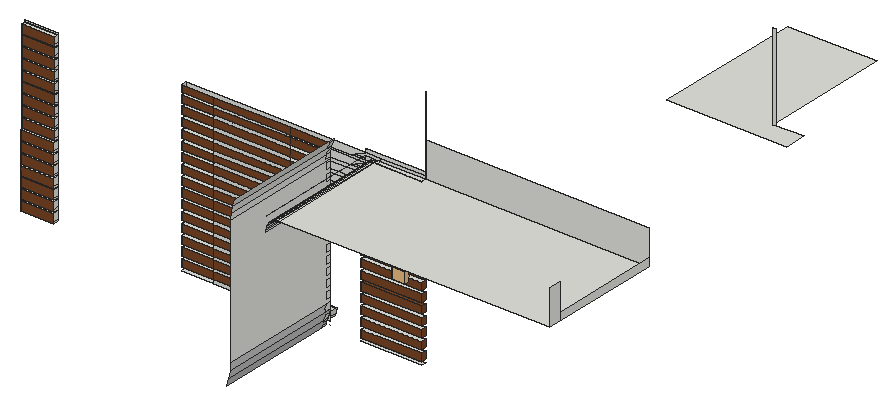
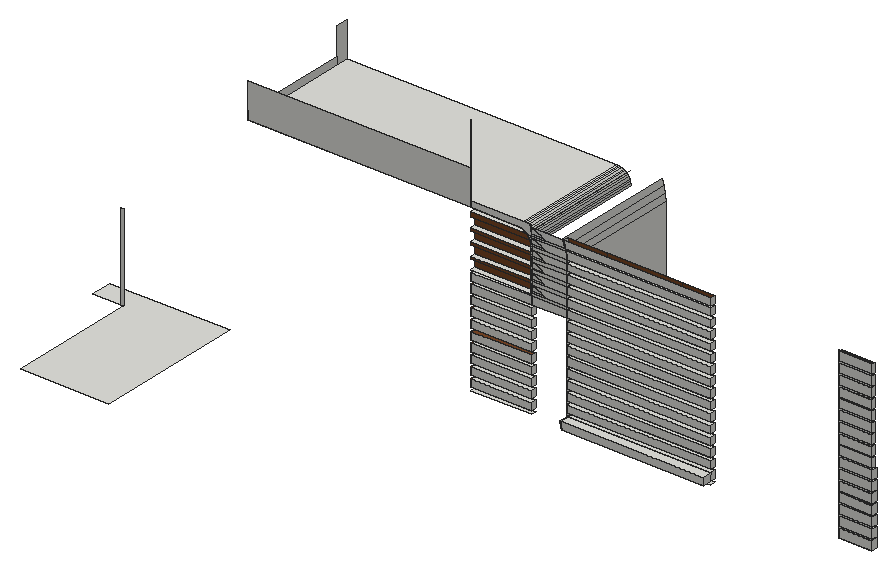
# SketchUp Ruby script. Lengths in inches.
U = 1.inch
M = Sketchup.active_model
def pt(a) = Geom::Point3d.new(a.map { |v| v * U })
def face(e, loops, mat)
  f = e.add_face(loops[0].map { |a| pt(a) })
  loops[1..].each { |l| e.add_face(l.map { |a| pt(a) }).erase! }
  f.material = f.back_material = mat if mat
  f
end
# faces: each face lists its corners as indices into pts; further lists are holes
def faces(e, pts, list, mat = nil) = list.each { |f| face(e, (f[0].is_a?(Array) ? f : [f]).map { |l| l.map { |i| pts[i] } }, mat) }
# xy, xz, yz: faces in a plane at the given z, y or x. An outline is a flat list of corners, or four numbers for a rectangle; further outlines are holes
def ring(l) = l.size == 4 ? [[l[0], l[1]], [l[2], l[1]], [l[2], l[3]], [l[0], l[3]]] : l.each_slice(2).to_a
def flat(e, list, mat, &to3) = list.each { |f| face(e, (f[0].is_a?(Array) ? f : [f]).map { |l| ring(l).map { |u, v| to3.(u, v) } }, mat) }
def xy(e, z, list, mat = nil) = flat(e, list, mat) { |x, y| [x, y, z] }
def xz(e, y, list, mat = nil) = flat(e, list, mat) { |x, z| [x, y, z] }
def yz(e, x, list, mat = nil) = flat(e, list, mat) { |y, z| [x, y, z] }
def lines(e, pts, list) = list.each { |a, b| e.add_line(pt(pts[a]), pt(pts[b])) }
# prism: a flat outline (further loops are holes) pulled along v
def prism(e, loops, v, mat = nil)
  f = face(e, loops, mat); d = Geom::Vector3d.new(v.map { |x| x * U })
  f.pushpull(f.normal.samedirection?(d) ? d.length : -d.length)
end
def box(e, o, s, mat = nil) = prism(e, [[o, [o[0] + s[0], o[1], o[2]], [o[0] + s[0], o[1] + s[1], o[2]], [o[0], o[1] + s[1], o[2]]]], [0, 0, s[2]], mat)
def at(x, y, z, deg = 0) = Geom::Transformation.translation(pt([x, y, z])) * Geom::Transformation.rotation(ORIGIN, Z_AXIS, deg.degrees)
def axes(o, x, y, z) = Geom::Transformation.new([*x, 0, *y, 0, *z, 0, *pt(o).to_a, 1])
def part(name) = M.definitions.add(name)
# library, detail: a bought-in or finely detailed component or shape, given as its bounding box
def library(name, o, s) = part(name).tap { |d| box(d.entities, o, s) }
def detail(e, o, s) = box(e.add_group.entities, o, s)
def put(e, d, t, mat = nil) = e.add_instance(d, t).tap { |i| i.material = mat if mat }
def group(e, t, mat = nil) = e.add_group.tap { |g| g.transformation = t; g.material = mat if mat }.entities
root = M.entities
M.materials.add("[Color M02]").color = [198, 198, 198]
M.materials.add("[Wood Veneer 01]").color = [120, 70, 37]
c1 = library("Spot+Bela",[0,3.21,0],[8.99,3.48,7.7])
xy(root,84.625,[[338.58,345.98,352.5,348.1]])
xy(root,85.73,[[405.46,345.98,463.86,348.1],[480.01,345.98,505.26,348.1]])
xy(root,87.0625,[[405.46,345.98,464.3125,348.1],[480.01,345.98,505.26,348.1],[405.46,348.1,464.3125,352.04]])
xy(root,88.34,[[338.58,345.98,352.5,348.1]])
xy(root,89,[[338.58,345.98,352.5,348.1]])
xy(root,90.11,[[405.46,345.98,465.05,348.1],[480.01,345.98,505.26,348.1],[405.46,348.1,465.05,352.04]])
xy(root,91.45,[[405.46,345.98,465.27,348.1],[480.01,345.98,505.26,348.1]])
xy(root,92.72,[[338.58,345.98,352.5,348.1]])
xy(root,93.375,[[338.58,345.98,352.5,348.1]])
xy(root,94.5,[[405.46,345.98,465.45,348.1],[480.01,345.98,505.26,348.1]])
xy(root,95.83,[[405.46,345.98,465.45,348.1],[480.01,345.98,505.26,348.1]])
xy(root,97.09,[[338.58,345.98,352.5,348.1]])
xy(root,97.75,[[338.58,345.98,352.5,348.1]])
xy(root,98.88,[[405.46,345.98,465.45,348.1],[480.01,345.98,505.26,348.1]])
xy(root,100.22,[[405.46,345.98,465.45,348.1],[480.01,345.98,505.26,348.1]])
xy(root,101.47,[[338.58,345.98,352.5,348.1]])
xy(root,102.125,[[338.58,345.98,352.5,348.1]])
xy(root,103.27,[[405.46,345.98,465.45,348.1],[480.01,345.98,505.26,348.1]])
xy(root,104.6,[[405.46,345.98,465.45,348.1],[480.01,345.98,505.26,348.1]])
xy(root,105.84,[[338.58,345.98,352.5,348.1]])
xy(root,106.5,[[338.58,345.98,352.5,348.1]])
xy(root,107.66,[[405.46,345.98,465.45,348.1]])
xy(root,107.66,[[480.01,345.98,505.26,348.1]],"[Wood Veneer 01]")
xy(root,108.99,[[405.46,345.98,465.45,348.1],[480.01,345.98,505.26,348.1]])
xy(root,110.22,[[338.58,345.98,352.5,348.1]])
xy(root,110.875,[[338.58,345.98,352.5,348.1]])
xy(root,112.04,[[405.46,345.98,465.45,348.1],[480.01,345.98,505.26,348.1]])
xy(root,113.375,[[405.46,345.98,465.45,348.1],[480.01,345.98,505.26,348.1]])
xy(root,114.59,[[338.58,345.98,352.5,348.1]])
xy(root,115.25,[[338.58,346.73,352.5,348.1]])
xy(root,116.43,[[405.46,345.98,465.45,348.1],[480.01,345.98,505.26,348.1]])
xy(root,117.76,[[405.46,345.98,465.45,348.1],[480.01,345.98,505.26,348.1]])
xy(root,118.97,[[338.58,346.73,352.5,348.1]])
xy(root,119.625,[[338.58,346.73,352.5,348.1]])
xy(root,120.8125,[[405.46,345.98,465.45,348.1],[480.01,345.98,505.26,348.1]])
xy(root,122.15,[[405.46,345.98,465.45,348.1],[480.01,345.98,505.26,348.1]])
xy(root,123.34,[[338.58,346.73,352.5,348.1]])
xy(root,124,[[338.58,346.73,352.5,348.1]])
xy(root,125.2,[[405.46,345.98,465.45,348.1],[480.01,345.98,505.26,348.1]])
xy(root,126.53,[[405.46,345.98,465.45,348.1],[480.01,345.98,505.26,348.1]])
xy(root,127.72,[[338.58,346.73,352.5,348.1]])
xy(root,128.375,[[338.58,346.73,352.5,348.1]])
xy(root,129.58,[[405.46,345.98,465.45,348.1],[480.01,345.98,505.26,348.1]])
xy(root,130.59,[[480.01,345.98,505.26,348.42]])
xy(root,130.92,[[405.48,345.98,465.45,348.1]])
xy(root,132.09,[[338.58,346.73,352.5,348.1]])
xy(root,132.75,[[338.58,346.73,352.5,348.1]])
xy(root,133.82,[[405.48,345.98,465.45,348.1]])
xy(root,134.72,[[480.01,345.98,505.26,348.42]])
xy(root,135.29,[[405.48,345.98,465.45,348.1]])
xy(root,135.72,[[480.01,345.98,505.26,348.42]])
xy(root,136.47,[[338.58,346.73,352.5,348.1]])
xy(root,137.125,[[338.58,346.73,352.5,348.1]])
xy(root,138.2,[[405.48,345.98,465.45,348.1]])
xy(root,139.67,[[405.48,345.98,465.45,348.1]])
xy(root,139.85,[[480.01,345.98,505.26,348.42]])
xy(root,140.84,[[338.58,346.73,352.5,348.1]])
xy(root,141.08,[[480.01,345.98,505.26,348.42]])
xy(root,141.5,[[338.58,346.73,352.5,348.1]])
xy(root,142.57,[[405.48,345.98,465.45,348.1]])
xy(root,144.04,[[405.48,345.98,465.45,348.1]])
xy(root,145.21,[[480.01,345.98,505.26,348.42]])
xy(root,145.22,[[338.58,346.73,352.5,348.1]])
xy(root,145.75,[[524.68,449.29,524.68,511.73,561.55,511.73,561.55,458.23,574.17,458.23,574.17,449.29]])
xy(root,145.875,[[338.58,346.73,352.5,348.1]])
xy(root,146.46,[[480.01,345.98,505.26,348.42]])
xy(root,146.95,[[405.48,345.98,465.45,348.1]])
xy(root,148.42,[[405.48,345.98,465.52,348.1]])
xy(root,149.59,[[338.58,346.73,352.5,348.1]])
xy(root,150.25,[[338.58,346.73,352.5,348.1]])
xy(root,150.58,[[480.57,345.98,505.26,348.42]])
xy(root,151.32,[[405.48,345.98,465.87,348.1]])
xy(root,152.17,[[405.48,345.98,466.04,348.1]])
xy(root,152.27,[[481.75,346.17,505.26,348.42]])
xy(root,153.97,[[485.86,296.73,485.86,346.17,505.26,346.17,505.26,348.1,597.79,348.1,597.79,296.73],[485.86,346.17,486.52,348.1],[486.52,346.17,505.26,348.1],[338.58,346.73,352.5,348.1],[485.86,348.1,486.52,348.42],
  [486.52,348.1,505.26,348.42]])
xz(root,345.98,[[419.16,85.73,450.71,87.0625],[419.16,90.11,450.71,91.45],[419.16,94.5,450.71,95.83],[419.16,98.88,450.71,100.22],[419.16,103.27,450.71,104.6],
  [419.16,107.66,450.71,108.99],[419.16,112.04,450.71,113.375],[419.16,116.43,450.71,117.76],[419.16,120.8125,450.71,122.15],[419.16,125.2,450.71,126.53],
  [419.16,129.58,450.71,130.92],[419.16,133.82,450.71,135.29],[419.16,138.2,450.71,139.67],[419.16,142.57,450.71,144.04],[419.16,146.95,450.71,148.42],
  [419.16,151.32,450.71,152.17]])
xz(root,345.98,[[338.58,84.625,352.5,88.34],[405.46,87.0625,419.16,90.11],[419.16,87.0625,450.71,90.11],[450.71,87.0625,464.3125,87.0625,464.64,88.01,465.05,90.11,450.71,90.11],[480.01,87.0625,505.26,90.11],
  [338.58,89,352.5,92.72],[405.46,91.45,419.16,94.5],[419.16,91.45,450.71,94.5],[450.71,91.45,465.27,91.45,465.45,94.23,465.45,94.5,450.71,94.5],[480.01,91.45,505.26,94.5],
  [338.58,93.375,352.5,97.09],[405.46,95.83,419.16,98.88],[419.16,95.83,450.71,98.88],[450.71,95.83,465.45,98.88],[480.01,95.83,505.26,98.88],
  [338.58,97.75,352.5,101.47],[405.46,100.22,419.16,103.27],[419.16,100.22,450.71,103.27],[450.71,100.22,465.45,103.27],[480.01,100.22,505.26,103.27],
  [338.58,102.125,352.5,105.84],[405.46,104.6,419.16,107.66],[419.16,104.6,450.71,107.66],[450.71,104.6,465.45,107.66],[480.01,104.6,505.26,107.66],
  [338.58,106.5,352.5,110.22],[405.46,108.99,419.16,112.04],[419.16,108.99,450.71,112.04],[450.71,108.99,465.45,112.04],[480.01,108.99,505.26,112.04],
  [338.58,110.875,352.5,114.59],[405.46,113.375,419.16,116.43],[419.16,113.375,450.71,116.43],[450.71,113.375,465.45,116.43],[480.01,113.375,505.26,116.43],
  [405.46,117.76,419.16,120.8125],[419.16,117.76,450.71,120.8125],[450.71,117.76,465.45,120.8125],[480.01,117.76,505.26,120.8125],[405.46,122.15,419.16,125.2],
  [419.16,122.15,450.71,125.2],[450.71,122.15,465.45,125.2],[480.01,122.15,505.26,125.2],[405.46,126.53,419.16,129.58],[419.16,126.53,450.71,129.58],
  [450.71,126.53,465.45,129.58],[480.01,126.53,505.26,129.58],[480.01,130.59,505.26,134.72],[405.48,130.92,419.16,133.82],[419.16,130.92,450.71,133.82],
  [450.71,130.92,465.45,133.82],[405.48,135.29,419.16,138.2],[419.16,135.29,450.71,138.2],[450.71,135.29,465.45,138.2],[480.01,135.72,505.26,139.85],
  [405.48,139.67,419.16,142.57],[419.16,139.67,450.71,142.57],[450.71,139.67,465.45,142.57],[480.01,141.08,505.26,145.21],[405.48,144.04,419.16,146.95],
  [419.16,144.04,450.71,146.95],[450.71,144.04,465.45,146.95],[480.01,146.46,505.26,146.46,505.26,150.58,480.57,150.58,480.45,150.35,480.21,149.63,480.06,148.88,480.01,148.12],[405.48,148.42,419.16,151.32],[419.16,148.42,450.71,151.32],
  [450.71,148.42,465.52,148.42,465.63,150.15,465.87,151.32,450.71,151.32],[405.48,152.17,419.16,155.07],[419.16,152.17,450.71,155.07],[450.71,152.17,466.04,152.17,466.17,152.85,466.92,155.07,450.71,155.07]],"[Wood Veneer 01]")
xz(root,346.17,[[481.75,152.27,505.26,152.27,505.26,153.97,485.86,153.97,485.09,153.92,484.34,153.77,483.62,153.52,482.93,153.18,482.3,152.76]],"[Wood Veneer 01]")
xz(root,346.73,[[338.58,115.25,352.5,118.97],[338.58,119.625,352.5,123.34],[338.58,124,352.5,127.72],[338.58,128.375,352.5,132.09],[338.58,132.75,352.5,136.47],
  [338.58,137.125,352.5,140.84],[338.58,141.5,352.5,145.22],[338.58,145.875,352.5,149.59],[338.58,150.25,352.5,153.97]],"[Wood Veneer 01]")
xz(root,348.1,[[338.58,84.625,352.5,88.34],[405.46,87.0625,405.46,90.11,465.05,90.11,464.64,88.01,464.3125,87.0625],[464.3125,87.0625,465.27,87.0625,465.45,89.84,465.45,90.11,465.05,90.11,464.64,88.01],[480.01,87.0625,505.26,90.11],[338.58,88.34,352.5,89],
  [338.58,89,352.5,92.72],[405.46,91.45,405.46,94.5,465.45,94.5,465.45,94.23,465.27,91.45],[465.27,91.45,465.45,91.45,465.45,94.23],[480.01,91.45,505.26,94.5],[338.58,92.72,352.5,93.375],
  [338.58,93.375,352.5,97.09],[405.46,95.83,465.45,98.88],[480.01,95.83,505.26,98.88],[338.58,97.09,352.5,97.75],[338.58,97.75,352.5,101.47],
  [405.46,100.22,465.45,103.27],[480.01,100.22,505.26,103.27],[338.58,101.47,352.5,102.125],[338.58,102.125,352.5,105.84],[405.46,104.6,465.45,107.66],
  [480.01,104.6,505.26,107.66],[338.58,105.84,352.5,106.5],[338.58,106.5,352.5,110.22],[405.46,108.99,465.45,112.04],[480.01,108.99,505.26,112.04],
  [338.58,110.22,352.5,110.875],[338.58,110.875,352.5,114.59],[405.46,113.375,465.45,116.43],[480.01,113.375,505.26,116.43],[338.58,114.59,352.5,115.25],
  [338.58,115.25,352.5,118.97],[405.46,117.76,465.45,120.8125],[480.01,117.76,505.26,120.8125],[338.58,118.97,352.5,119.625],[338.58,119.625,352.5,123.34],
  [405.46,122.15,465.45,125.2],[480.01,122.15,505.26,125.2],[338.58,123.34,352.5,124],[338.58,124,352.5,127.72],[405.46,126.53,465.45,129.58],
  [465.45,126.53,480.01,129.58],[480.01,126.53,505.26,129.58],[338.58,127.72,352.5,128.375],[338.58,128.375,352.5,132.09],[465.45,129.58,480.01,130.92],
  [405.48,130.92,465.45,133.82],[465.45,130.92,474.62,130.92,475.625,131.59,475.99,131.83,478.46,133.05,480.01,133.58,480.01,133.82,465.45,133.82],[474.62,130.92,480.01,130.92,480.01,131.59,475.625,131.59],[475.625,131.59,480.01,131.59,480.01,133.58,478.46,133.05,475.99,131.83],[338.58,132.09,352.5,132.75],
  [338.58,132.75,352.5,136.47],[465.45,133.82,480.01,135.29],[405.48,135.29,465.45,138.2],[465.45,135.29,474.62,135.29,475.625,135.97,475.99,136.21,478.46,137.42,480.01,137.95,480.01,138.2,465.45,138.2],[474.62,135.29,480.01,135.29,480.01,135.97,475.625,135.97],
  [475.625,135.97,480.01,135.97,480.01,137.95,478.46,137.42,475.99,136.21],[338.58,136.47,352.5,137.125],[338.58,137.125,352.5,140.84],[465.45,138.2,480.01,139.67],[405.48,139.67,465.45,142.57],
  [465.45,139.67,474.62,139.67,475.625,140.34,475.99,140.58,478.46,141.8,480.01,142.33,480.01,142.57,465.45,142.57],[474.62,139.67,480.01,139.67,480.01,140.34,475.625,140.34],[475.625,140.34,480.01,140.34,480.01,142.33,478.46,141.8,475.99,140.58],[338.58,140.84,352.5,141.5],[338.58,141.5,352.5,145.22],
  [465.45,142.57,480.01,144.04],[405.48,144.04,465.45,146.95],[465.45,144.04,474.62,144.04,475.625,144.72,475.99,144.96,478.46,146.17,480.01,146.7,480.01,146.95,465.45,146.95],[474.62,144.04,480.01,144.04,480.01,144.72,475.625,144.72],[475.625,144.72,480.01,144.72,480.01,146.7,478.46,146.17,475.99,144.96],
  [338.58,145.22,352.5,145.875],[338.58,145.875,352.5,149.59],[465.45,146.95,480.01,146.95,480.01,148.42,465.52,148.42,465.45,147.4],[405.48,148.42,405.48,151.32,465.87,151.32,465.63,150.15,465.52,148.42],[465.52,148.42,474.62,148.42,475.625,149.09,475.99,149.33,478.46,150.55,480.01,151.08,480.01,151.32,465.87,151.32,465.63,150.15],
  [474.62,148.42,480.01,148.42,480.01,149.09,475.625,149.09],[475.625,149.09,480.01,149.09,480.01,151.08,478.46,150.55,475.99,149.33],[338.58,149.59,352.5,150.25],[338.58,150.25,352.5,153.97],[465.87,151.32,480.01,151.32,480.01,152.17,466.04,152.17],
  [405.48,152.17,405.48,155.07,466.92,155.07,466.17,152.85,466.04,152.17],[466.04,152.17,474.62,152.17,475.625,152.84,475.99,153.08,478.46,154.3,480.73,155.07,466.92,155.07,466.17,152.85],[474.62,152.17,480.01,152.17,480.01,152.84,475.625,152.84],[475.625,152.84,480.01,152.84,480.01,153.97,486.52,153.97,486.52,155.07,480.73,155.07,478.46,154.3,475.99,153.08],[338.58,153.97,352.5,154.625],
  [486.52,153.97,505.26,155.07],[505.26,153.97,597.79,168.47]])
xz(root,348.42,[[480.01,148.12,480.06,148.88,480.21,149.63,480.45,150.35,480.57,150.58,480.01,150.58],[480.01,152.27,481.75,152.27,482.3,152.76,482.93,153.18,483.62,153.52,484.34,153.77,485.09,153.92,485.86,153.97,505.26,153.97,505.26,156.4,480.57,156.4,480.45,156.17,480.21,155.45,480.06,154.7,480.01,153.9375],[480.01,153.9375,480.06,154.7,480.21,155.45,480.45,156.17,480.57,156.4,480.01,156.4]])
xz(root,348.42,[[480.01,134.72,505.26,135.72],[480.01,139.85,505.26,141.08],[480.01,145.21,505.26,146.46],[480.57,150.58,505.26,150.58,505.26,152.27,481.75,152.27,481.72,152.25,481.22,151.68,480.79,151.04]],"[Wood Veneer 01]")
xz(root,352.04,[[405.46,87.0625,405.46,90.11,465.05,90.11,464.64,88.01,464.3125,87.0625]])
xz(root,458.23,[[561.55,145.75,562.67,181.75]])
yz(root,338.58,[[345.98,84.625,348.1,88.34],[345.98,89,348.1,92.72],[345.98,93.375,348.1,97.09],[345.98,97.75,348.1,101.47],[345.98,102.125,348.1,105.84],
  [345.98,106.5,348.1,110.22],[345.98,110.875,348.1,114.59],[346.73,115.25,348.1,118.97],[346.73,119.625,348.1,123.34],[346.73,124,348.1,127.72],
  [346.73,128.375,348.1,132.09],[346.73,132.75,348.1,136.47],[346.73,137.125,348.1,140.84],[346.73,141.5,348.1,145.22],[346.73,145.875,348.1,149.59],
  [346.73,150.25,348.1,153.97]])
yz(root,352.5,[[345.98,84.625,348.1,85.5],[345.98,85.5,348.1,88.34],[345.98,89,348.1,89.875],[345.98,89.875,348.1,92.72],[345.98,93.375,348.1,94.25],
  [345.98,94.25,348.1,97.09],[345.98,97.75,348.1,98.625],[345.98,98.625,348.1,101.47],[345.98,102.125,348.1,103],[345.98,103,348.1,105.84],
  [345.98,106.5,348.1,107.375],[345.98,107.375,348.1,110.22],[345.98,110.875,348.1,111.75],[345.98,111.75,348.1,114.59],[346.73,115.25,348.1,116.125],
  [346.73,116.125,348.1,118.97],[346.73,119.625,348.1,120.5],[346.73,120.5,348.1,123.34],[346.73,124,348.1,124.875],[346.73,124.875,348.1,127.72],
  [346.73,128.375,348.1,129.25],[346.73,129.25,348.1,132.09],[346.73,132.75,348.1,133.625],[346.73,133.625,348.1,136.47],[346.73,137.125,348.1,138],
  [346.73,138,348.1,140.84],[346.73,141.5,348.1,142.375],[346.73,142.375,348.1,145.22],[346.73,145.875,348.1,146.75],[346.73,146.75,348.1,149.59],
  [346.73,150.25,348.1,151.125],[346.73,151.125,348.1,153.97]])
yz(root,405.46,[[345.98,87.0625,348.1,90.11],[348.1,87.0625,352.04,90.11],[345.98,91.45,348.1,94.5],[345.98,95.83,348.1,98.88],[345.98,100.22,348.1,103.27],
  [345.98,104.6,348.1,107.66],[345.98,108.99,348.1,112.04],[345.98,113.375,348.1,116.43],[345.98,117.76,348.1,120.8125],[345.98,122.15,348.1,125.2],
  [345.98,126.53,348.1,129.58]])
yz(root,405.48,[[345.98,130.92,348.1,133.82],[345.98,135.29,348.1,138.2],[345.98,139.67,348.1,142.57],[345.98,144.04,348.1,146.95],[345.98,148.42,348.1,151.32],
  [345.98,152.17,348.1,155.07]])
yz(root,465.45,[[296.73,94.23,296.73,147.4,348.1,147.4,348.1,146.95,345.98,146.95,345.98,144.04,348.1,144.04,348.1,142.57,345.98,142.57,345.98,139.67,348.1,139.67,348.1,138.2,345.98,138.2,345.98,135.29,348.1,135.29,348.1,133.82,345.98,133.82,345.98,130.92,348.1,130.92,348.1,129.58,345.98,129.58,345.98,126.53,348.1,126.53,348.1,125.2,345.98,125.2,345.98,122.15,348.1,122.15,348.1,120.8125,345.98,120.8125,345.98,117.76,348.1,117.76,348.1,116.43,345.98,116.43,345.98,113.375,348.1,113.375,348.1,112.04,345.98,112.04,345.98,108.99,348.1,108.99,348.1,107.66,345.98,107.66,345.98,104.6,348.1,104.6,348.1,103.27,345.98,103.27,345.98,100.22,348.1,100.22,348.1,98.88,345.98,98.88,345.98,95.83,348.1,95.83,348.1,94.5,345.98,94.5,345.98,94.23],[345.98,94.23,348.1,94.5],[345.98,95.83,348.1,98.88],[345.98,100.22,348.1,103.27],[345.98,104.6,348.1,107.66],
  [345.98,108.99,348.1,112.04],[345.98,113.375,348.1,116.43],[345.98,117.76,348.1,120.8125],[345.98,122.15,348.1,125.2],[345.98,126.53,348.1,129.58],
  [345.98,130.92,348.1,133.82],[345.98,135.29,348.1,138.2],[345.98,139.67,348.1,142.57],[345.98,144.04,348.1,146.95]])
yz(root,480.01,[[345.98,87.0625,348.1,90.11],[345.98,91.45,348.1,94.5],[345.98,95.83,348.1,98.88],[345.98,100.22,348.1,103.27],[345.98,104.6,348.1,107.66],
  [345.98,108.99,348.1,112.04],[345.98,113.375,348.1,116.43],[345.98,117.76,348.1,120.8125],[345.98,122.15,348.1,125.2],[345.98,126.53,348.1,129.58],
  [345.98,130.59,348.1,134.72],[348.1,130.59,348.42,134.72],[348.1,134.72,348.42,135.72],[345.98,135.72,348.1,139.85],[348.1,135.72,348.42,139.85],
  [348.1,139.85,348.42,141.08],[345.98,141.08,348.1,145.21],[348.1,141.08,348.42,145.21],[348.1,145.21,348.42,146.46],[345.98,146.46,348.1,148.12],
  [348.1,146.46,348.42,148.12]])
yz(root,505.26,[[348.1,153.97,348.42,186.3125]])
yz(root,505.26,[[345.98,87.0625,348.1,90.11],[345.98,91.45,348.1,94.5],[345.98,95.83,348.1,98.88],[345.98,100.22,348.1,103.27],[345.98,104.6,348.1,107.66],
  [345.98,108.99,348.1,112.04],[345.98,113.375,348.1,116.43],[345.98,117.76,348.1,120.8125],[345.98,122.15,348.1,125.2],[345.98,126.53,348.1,129.58]],"[Wood Veneer 01]")
yz(root,597.79,[[296.73,153.97,301.92,168.47],[301.92,153.97,348.1,157.09]])
p = [[463.625,296.73,85.04],[464.64,296.73,88.01],[464.64,345.98,88.01],[464.3125,345.98,87.0625],[464.3125,348.1,87.0625],[463.86,348.1,85.73],
  [463.86,345.98,85.73],[463.625,345.98,85.04],[463.625,348.1,85.04],[464.64,348.1,88.01],[464.3125,352.04,87.0625],[464.64,352.04,88.01],
  [465.25,296.73,91.1],[465.25,348.1,91.1],[465.05,348.1,90.11],[465.05,345.98,90.11],[465.05,352.04,90.11],[465.45,296.73,94.23],
  [465.45,345.98,94.23],[465.27,345.98,91.45],[465.27,348.1,91.45],[465.45,348.1,94.23],[465.45,296.73,147.4],[465.63,296.73,150.15],
  [465.63,345.98,150.15],[465.52,345.98,148.42],[465.52,348.1,148.42],[465.45,348.1,147.4],[480.06,296.73,148.88],[480.01,296.73,148.12],
  [480.01,345.98,148.12],[480.06,345.98,148.88],[480.01,348.42,148.12],[480.06,348.42,148.88],[480.01,348.1,148.12],[465.63,348.1,150.15],
  [480.21,296.73,149.63],[480.21,345.98,149.63],[480.21,348.42,149.63],[480.45,296.73,150.35],[480.45,345.98,150.35],[480.45,348.42,150.35],
  [466.17,296.73,152.85],[466.17,345.98,152.85],[466.04,345.98,152.17],[466.04,348.1,152.17],[465.87,348.1,151.32],[465.87,345.98,151.32],
  [480.79,296.73,151.04],[480.57,345.98,150.58],[480.57,348.42,150.58],[480.79,348.42,151.04],[481.22,296.73,151.68],[481.22,348.42,151.68],
  [481.72,296.73,152.25],[481.72,348.42,152.25],[466.17,348.1,152.85],[482.3,296.73,152.76],[481.75,348.42,152.27],[481.75,346.17,152.27],
  [482.3,346.17,152.76],[482.3,348.42,152.76],[482.93,296.73,153.18],[482.93,346.17,153.18],[482.93,348.42,153.18],[467.06,296.73,155.46],
  [467.06,348.1,155.46],[466.92,348.1,155.07],[466.92,345.98,155.07],[483.62,296.73,153.52],[483.62,346.17,153.52],[483.62,348.42,153.52],
  [484.34,296.73,153.77],[484.34,346.17,153.77],[484.34,348.42,153.77],[485.09,296.73,153.92],[485.09,346.17,153.92],[485.09,348.42,153.92],
  [485.86,296.73,153.97],[485.86,346.17,153.97],[485.86,348.42,153.97],[485.86,348.1,153.97],[480.01,296.73,153.97],[480.01,348.1,153.97],
  [480.73,348.1,151.32],[480.01,348.1,151.08],[480.01,348.1,151.32],[480.73,348.1,146.95],[480.01,348.1,146.7],[480.01,348.1,146.95],
  [480.73,348.1,142.57],[480.01,348.1,142.33],[480.01,348.1,142.57],[480.73,348.1,138.2],[480.01,348.1,138.2],[480.01,348.1,137.95],
  [480.73,348.1,133.82],[480.01,348.1,133.58],[480.01,348.1,133.82],[465.45,348.1,87.0625],[465.27,348.1,87.0625],[465.05,348.1,85.73],
  [465.45,348.1,85.73]]
faces(root,p,[[0,1,2,3,4,5,6,7],[1,12,13,14,15,2],[12,17,18,19,20,13]],"[Color M02]")
faces(root,p,[[5,8,7,6],[9,4,3,2],[9,4,10,11],[14,9,2,15],[14,9,11,16],[21,20,19,18],[22,23,24,25,26,27],[28,29,30,31],
  [32,33,31,30,34],[35,26,25,24],[36,28,31,37],[33,38,37,31],[39,36,37,40],[38,41,40,37],[23,42,43,44,45,46,47,24],[46,35,24,47],
  [48,39,40,49,50,51],[41,50,49,40],[52,48,51,53],[54,52,53,55],[56,45,44,43],[57,54,55,58,59,60],[58,61,60,59],[62,57,60,63],
  [61,64,63,60],[42,65,66,67,68,43],[67,56,43,68],[69,62,63,70],[64,71,70,63],[72,69,70,73],[71,74,73,70],[75,72,73,76],
  [74,77,76,73],[78,75,76,79],[77,80,81,79,76]])
lines(root,p,[[82,83],[84,85],[84,86],[87,88],[87,89],[90,91],[90,92],[93,94],[93,95],[96,97],[96,98],[99,100],
  [101,102]])
put(root,c1,axes([494.42,342.07,114.71],[0.59,0,0],[0,0.59,0],[0,0,0.59]))
